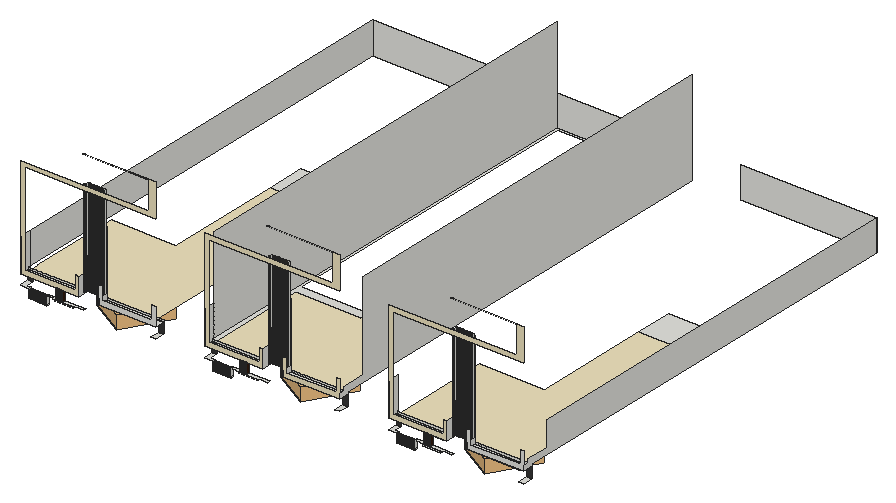
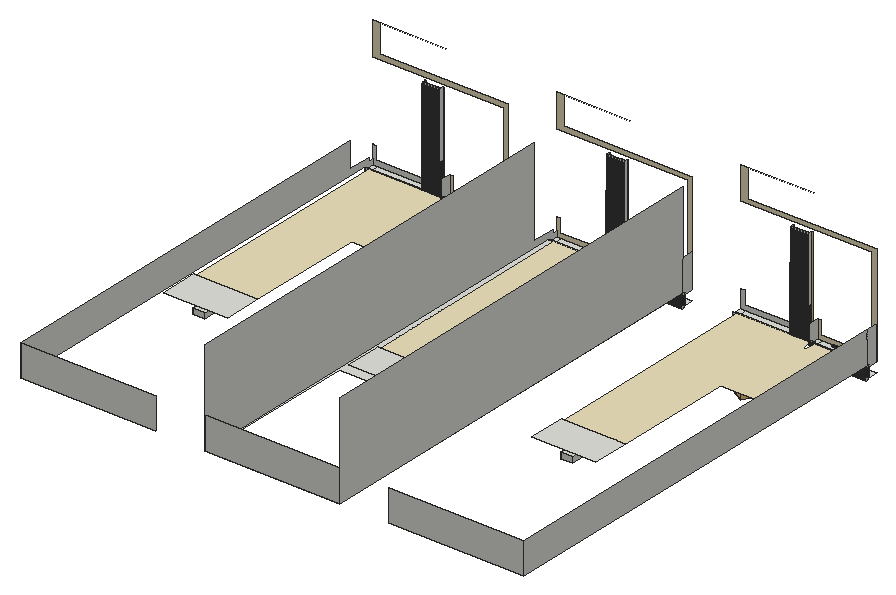
# SketchUp Ruby script. Lengths in inches.
U = 1.inch
M = Sketchup.active_model
def pt(a) = Geom::Point3d.new(a.map { |v| v * U })
def face(e, loops, mat)
  f = e.add_face(loops[0].map { |a| pt(a) })
  loops[1..].each { |l| e.add_face(l.map { |a| pt(a) }).erase! }
  f.material = f.back_material = mat if mat
  f
end
# faces: each face lists its corners as indices into pts; further lists are holes
def faces(e, pts, list, mat = nil) = list.each { |f| face(e, (f[0].is_a?(Array) ? f : [f]).map { |l| l.map { |i| pts[i] } }, mat) }
# xy, xz, yz: faces in a plane at the given z, y or x. An outline is a flat list of corners, or four numbers for a rectangle; further outlines are holes
def ring(l) = l.size == 4 ? [[l[0], l[1]], [l[2], l[1]], [l[2], l[3]], [l[0], l[3]]] : l.each_slice(2).to_a
def flat(e, list, mat, &to3) = list.each { |f| face(e, (f[0].is_a?(Array) ? f : [f]).map { |l| ring(l).map { |u, v| to3.(u, v) } }, mat) }
def xy(e, z, list, mat = nil) = flat(e, list, mat) { |x, y| [x, y, z] }
def xz(e, y, list, mat = nil) = flat(e, list, mat) { |x, z| [x, y, z] }
def yz(e, x, list, mat = nil) = flat(e, list, mat) { |y, z| [x, y, z] }
def lines(e, pts, list) = list.each { |a, b| e.add_line(pt(pts[a]), pt(pts[b])) }
# prism: a flat outline (further loops are holes) pulled along v
def prism(e, loops, v, mat = nil)
  f = face(e, loops, mat); d = Geom::Vector3d.new(v.map { |x| x * U })
  f.pushpull(f.normal.samedirection?(d) ? d.length : -d.length)
end
def box(e, o, s, mat = nil) = prism(e, [[o, [o[0] + s[0], o[1], o[2]], [o[0] + s[0], o[1] + s[1], o[2]], [o[0], o[1] + s[1], o[2]]]], [0, 0, s[2]], mat)
def at(x, y, z, deg = 0) = Geom::Transformation.translation(pt([x, y, z])) * Geom::Transformation.rotation(ORIGIN, Z_AXIS, deg.degrees)
def axes(o, x, y, z) = Geom::Transformation.new([*x, 0, *y, 0, *z, 0, *pt(o).to_a, 1])
def part(name) = M.definitions.add(name)
# library, detail: a bought-in or finely detailed component or shape, given as its bounding box
def library(name, o, s) = part(name).tap { |d| box(d.entities, o, s) }
def detail(e, o, s) = box(e.add_group.entities, o, s)
def put(e, d, t, mat = nil) = e.add_instance(d, t).tap { |i| i.material = mat if mat }
def group(e, t, mat = nil) = e.add_group.tap { |g| g.transformation = t; g.material = mat if mat }.entities
root = M.entities
M.materials.add("[Color D01]").color = [237, 225, 189]
M.materials.add("[Slate Light Tile]").color = [54, 54, 54]
M.materials.add("[Slate]").color = [102, 110, 108]
M.materials.add("[Wood Veneer 01]").color = [51, 28, 15]
c1 = library("002+Bmw+M4+++mat3.4+2017",[-252.8,19.48,9.01],[196.94,171.32,55.15])
c2 = library("Group\#1",[-0.5,-0.5,0],[4.42,1,384])
c3 = library("Group\#4",[-0.5,-0.5,0],[4.42,1,384])
xy(root,44.76,[[115.73,246.64,188.54,248.89],[849.29,246.64,922.1,248.89],[1582.85,246.64,1655.66,248.89],[115.73,248.89,188.54,254.15],[188.54,248.89,190.1,254.15],
  [849.29,248.89,922.1,254.15],[922.1,248.89,923.66,254.15],[1582.85,248.89,1655.66,254.15],[1655.66,248.89,1657.23,254.15],[115.73,254.15,188.54,255.71],
  [849.29,254.15,922.1,255.71],[1582.85,254.15,1655.66,255.71]])
xy(root,47.875,[[115.73,248.89,190.1,254.15],[849.29,248.89,923.66,254.15],[1582.85,248.89,1657.23,254.15]])
xy(root,50.625,[[115.73,248.89,188.54,254.15],[849.29,248.89,922.1,254.15],[1582.85,248.89,1655.66,254.15]])
xy(root,53.875,[[115.73,248.89,188.54,254.15],[849.29,248.89,922.1,254.15],[1582.85,248.89,1655.66,254.15]])
xy(root,56.625,[[115.73,248.89,188.54,254.15],[849.29,248.89,922.1,254.15],[1582.85,248.89,1655.66,254.15]])
xy(root,59.875,[[115.73,248.89,188.54,254.15],[849.29,248.89,922.1,254.15],[1582.85,248.89,1655.66,254.15]])
xy(root,62.625,[[115.73,248.89,188.54,254.15],[849.29,248.89,922.1,254.15],[1582.85,248.89,1655.66,254.15]])
xy(root,65.875,[[115.73,248.89,188.54,254.15],[849.29,248.89,922.1,254.15],[1582.85,248.89,1655.66,254.15]])
xy(root,68.625,[[115.73,248.89,188.54,254.15],[849.29,248.89,922.1,254.15],[1582.85,248.89,1655.66,254.15]])
xy(root,71.875,[[115.73,248.89,188.54,254.15],[849.29,248.89,922.1,254.15],[1582.85,248.89,1655.66,254.15]])
xy(root,74.24,[[224.55,243.46,295.95,246.64],[958.11,243.46,1029.51,246.64],[1691.68,243.46,1763.07,246.64]])
xy(root,74.625,[[115.73,248.89,188.54,254.15],[849.29,248.89,922.1,254.15],[1582.85,248.89,1655.66,254.15]])
xy(root,76.4375,[[603.24,246.64,622,286.21],[1336.8,246.64,1355.5625,286.21],[2070.36,246.64,2089.125,286.21]])
xy(root,77.875,[[115.73,248.89,188.54,254.15],[849.29,248.89,922.1,254.15],[1582.85,248.89,1655.66,254.15]])
xy(root,79.95,[[215.84,243.46,224.54,243.46,224.54,255.71,188.54,255.71,188.54,246.64,215.84,246.64],[224.54,243.46,230.14,246.64],[230.14,243.46,235.97,246.64],[235.97,243.46,241.57,246.64],[241.57,243.46,248.39,246.64],
  [248.39,243.46,253.99,246.64],[253.99,243.46,303.85,243.46,303.85,246.64,337.76,246.64,337.76,255.71,253.99,255.71],[949.4,243.46,958.1,243.46,958.1,255.71,922.1,255.71,922.1,246.64,949.4,246.64],[958.1,243.46,963.7,246.64],[963.7,243.46,969.54,246.64],
  [969.54,243.46,975.14,246.64],[975.14,243.46,981.95,246.64],[981.95,243.46,987.55,246.64],[987.55,243.46,1037.42,243.46,1037.42,246.64,1071.32,246.64,1071.32,255.71,987.55,255.71],[1682.97,243.46,1691.67,243.46,1691.67,255.71,1655.66,255.71,1655.66,246.64,1682.97,246.64],
  [1691.67,243.46,1697.27,246.64],[1697.27,243.46,1703.1,246.64],[1703.1,243.46,1708.7,246.64],[1708.7,243.46,1715.51,246.64],[1715.51,243.46,1721.11,246.64],
  [1721.11,243.46,1770.98,243.46,1770.98,246.64,1804.89,246.64,1804.89,255.71,1721.11,255.71],[83.125,246.64,115.73,246.64,115.73,255.71,101.95,255.71,101.95,286.21,83.125,286.21],[230.14,246.64,235.97,255.71],[241.57,246.64,248.39,255.71],[816.6875,246.64,849.29,246.64,849.29,255.71,835.51,255.71,835.51,286.21,816.6875,286.21],
  [963.7,246.64,969.54,255.71],[975.14,246.64,981.95,255.71],[1550.25,246.64,1582.85,246.64,1582.85,255.71,1569.07,255.71,1569.07,286.21,1550.25,286.21],[1697.27,246.64,1703.1,255.71],[1708.7,246.64,1715.51,255.71]])
xy(root,79.95,[[224.54,246.64,230.14,255.71],[235.97,246.64,241.57,255.71],[248.39,246.64,253.99,255.71],[958.1,246.64,963.7,255.71],[969.54,246.64,975.14,255.71],
  [981.95,246.64,987.55,255.71],[1691.67,246.64,1697.27,255.71],[1703.1,246.64,1708.7,255.71],[1715.51,246.64,1721.11,255.71]],"[Wood Veneer 01]")
xy(root,91.5625,[[452.08,1150.15,500.08,1298.96],[1185.65,1150.15,1233.65,1298.96],[1919.21,1150.15,1967.21,1298.96]])
xy(root,114.3125,[[452.08,1150.15,500.08,1298.96],[1185.65,1150.15,1233.65,1298.96],[1919.21,1150.15,1967.21,1298.96]])
xy(root,120.375,[[83.125,246.64,83.125,286.21,298.48,286.21,298.48,246.64,253.99,246.64,253.99,255.71,248.39,255.71,248.39,246.64,241.57,246.64,241.57,255.71,235.97,255.71,235.97,246.64,230.14,246.64,230.14,255.71,224.54,255.71,224.54,246.64],[298.48,246.64,315.43,286.21],[396.57,246.64,603.24,286.21],[603.24,246.64,622,286.21],[816.6875,246.64,816.6875,286.21,1032.04,286.21,1032.04,246.64,987.55,246.64,987.55,255.71,981.95,255.71,981.95,246.64,975.14,246.64,975.14,255.71,969.54,255.71,969.54,246.64,963.7,246.64,963.7,255.71,958.1,255.71,958.1,246.64],
  [1032.04,246.64,1049,286.21],[1130.14,246.64,1336.8,286.21],[1336.8,246.64,1355.5625,286.21],[1550.25,246.64,1550.25,286.21,1765.6,286.21,1765.6,246.64,1721.11,246.64,1721.11,255.71,1715.51,255.71,1715.51,246.64,1708.7,246.64,1708.7,255.71,1703.1,255.71,1703.1,246.64,1697.27,246.64,1697.27,255.71,1691.67,255.71,1691.67,246.64],[1765.6,246.64,1782.56,286.21],
  [1863.7,246.64,2070.36,286.21],[2070.36,246.64,2089.125,286.21],[83.125,286.21,298.48,293.46],[298.48,286.21,315.43,293.46],[816.6875,286.21,1032.04,293.46],
  [1032.04,286.21,1049,293.46],[1550.25,286.21,1765.6,293.46],[1765.6,286.21,1782.56,293.46]])
xy(root,128.6875,[[[816.6875,286.21,816.6875,2003.89,1355.5625,2003.89,1355.5625,286.21,1336.8,286.21,1336.8,1150.15,1346.93,1150.15,1346.93,1298.96,1092.25,1298.96,1092.25,679.27,833.39,679.27,833.39,310.87,835.51,310.87,835.51,286.21],[825.32,714.9,1077.64,714.9,1077.64,1340.4,1346.93,1340.4,1346.93,1995.26,825.32,1995.26]],[358.6875,1150.15,613.36,1298.96],[1092.25,1150.15,1346.93,1298.96],[1825.8125,1150.15,2080.49,1298.96]])
xy(root,128.6875,[[[318.81,271.96,318.81,286.21,101.95,286.21,101.95,310.87,99.82,310.87,99.82,679.27,358.6875,679.27,358.6875,1150.15,603.24,1150.15,603.24,286.21,393.55,286.21,393.55,272.89,390.12,272.89,390.12,286.21,388.23,286.21,388.23,283.46,384.81,283.46,384.81,286.21,382.23,286.21,382.23,283.46,378.81,283.46,378.81,286.21,376.23,286.21,376.23,283.46,372.81,283.46,372.81,286.21,370.23,286.21,370.23,283.46,366.81,283.46,366.81,286.21,364.23,286.21,364.23,283.46,360.81,283.46,360.81,286.21,358.23,286.21,358.23,283.46,354.81,283.46,354.81,286.21,352.23,286.21,352.23,283.46,348.81,283.46,348.81,286.21,346.23,286.21,346.23,282.52,342.81,282.52,342.81,286.21,340.23,286.21,340.23,282.52,336.81,282.52,336.81,286.21,334.23,286.21,334.23,282.52,330.81,282.52,330.81,286.21,328.23,286.21,328.23,282.52,324.81,282.52,324.81,286.21,322.23,286.21,322.23,271.96],[294.56,294.84,310.12,329.78]],[[1052.37,271.96,1052.37,286.21,835.51,286.21,835.51,310.87,833.39,310.87,833.39,679.27,1092.25,679.27,1092.25,1150.15,1336.8,1150.15,1336.8,286.21,1127.11,286.21,1127.11,272.89,1123.68,272.89,1123.68,286.21,1121.8,286.21,1121.8,283.46,1118.37,283.46,1118.37,286.21,1115.8,286.21,1115.8,283.46,1112.37,283.46,1112.37,286.21,1109.8,286.21,1109.8,283.46,1106.37,283.46,1106.37,286.21,1103.8,286.21,1103.8,283.46,1100.37,283.46,1100.37,286.21,1097.8,286.21,1097.8,283.46,1094.37,283.46,1094.37,286.21,1091.8,286.21,1091.8,283.46,1088.37,283.46,1088.37,286.21,1085.8,286.21,1085.8,283.46,1082.37,283.46,1082.37,286.21,1079.8,286.21,1079.8,282.52,1076.37,282.52,1076.37,286.21,1073.8,286.21,1073.8,282.52,1070.37,282.52,1070.37,286.21,1067.8,286.21,1067.8,282.52,1064.37,282.52,1064.37,286.21,1061.8,286.21,1061.8,282.52,1058.37,282.52,1058.37,286.21,1055.8,286.21,1055.8,271.96],[1028.12,294.84,1043.68,329.78]],[[1785.93,271.96,1785.93,286.21,1569.07,286.21,1569.07,310.87,1566.95,310.87,1566.95,679.27,1825.8125,679.27,1825.8125,1150.15,2070.36,1150.15,2070.36,286.21,1860.67,286.21,1860.67,272.89,1857.25,272.89,1857.25,286.21,1855.36,286.21,1855.36,283.46,1851.93,283.46,1851.93,286.21,1849.36,286.21,1849.36,283.46,1845.93,283.46,1845.93,286.21,1843.36,286.21,1843.36,283.46,1839.93,283.46,1839.93,286.21,1837.36,286.21,1837.36,283.46,1833.93,283.46,1833.93,286.21,1831.36,286.21,1831.36,283.46,1827.93,283.46,1827.93,286.21,1825.36,286.21,1825.36,283.46,1821.93,283.46,1821.93,286.21,1819.36,286.21,1819.36,283.46,1815.93,283.46,1815.93,286.21,1813.36,286.21,1813.36,282.52,1809.93,282.52,1809.93,286.21,1807.36,286.21,1807.36,282.52,1803.93,282.52,1803.93,286.21,1801.36,286.21,1801.36,282.52,1797.93,282.52,1797.93,286.21,1795.36,286.21,1795.36,282.52,1791.93,282.52,1791.93,286.21,1789.36,286.21,1789.36,271.96],[1761.68,294.84,1777.24,329.78]]],"[Color D01]")
xz(root,246.64,[[396.57,120.375,622,120.375,622,193,609.07,193,609.07,140.625,409.32,140.625,409.32,193,396.57,193],[1863.7,120.375,2089.125,120.375,2089.125,193,2076.2,193,2076.2,140.625,1876.45,140.625,1876.45,193,1863.7,193]])
xz(root,246.64,[[83.125,120.375,315.43,120.375,315.43,193,303.35,193,303.35,140.625,100.18,140.625,100.18,506.8125,622,506.8125,622,636.53,330.81,636.53,330.81,635.84,593.4375,635.84,593.4375,524.9375,83.125,524.9375],[816.6875,120.375,1049,120.375,1049,193,1036.91,193,1036.91,140.625,833.74,140.625,833.74,506.8125,1355.5625,506.8125,1355.5625,636.53,1064.37,636.53,1064.37,635.84,1327,635.84,1327,524.9375,816.6875,524.9375],[1130.14,120.375,1355.5625,120.375,1355.5625,193,1342.64,193,1342.64,140.625,1142.89,140.625,1142.89,193,1130.14,193],[1550.25,120.375,1782.56,120.375,1782.56,193,1770.48,193,1770.48,140.625,1567.3,140.625,1567.3,506.8125,2089.125,506.8125,2089.125,636.53,1797.93,636.53,1797.93,635.84,2060.5625,635.84,2060.5625,524.9375,1550.25,524.9375]],"[Color D01]")
xz(root,246.64,[[230.14,79.95,235.97,120.375],[241.57,79.95,248.39,120.375],[963.7,79.95,969.54,120.375],[975.14,79.95,981.95,120.375],[1697.27,79.95,1703.1,120.375],
  [1708.7,79.95,1715.51,120.375]],"[Slate]")
xz(root,246.64,[[224.54,79.95,230.14,120.375],[235.97,79.95,241.57,120.375],[248.39,79.95,253.99,120.375],[958.1,79.95,963.7,120.375],[969.54,79.95,975.14,120.375],
  [981.95,79.95,987.55,120.375],[1691.67,79.95,1697.27,120.375],[1703.1,79.95,1708.7,120.375],[1715.51,79.95,1721.11,120.375]],"[Wood Veneer 01]")
xz(root,248.89,[[115.73,44.76,190.1,47.875],[849.29,44.76,923.66,47.875],[1582.85,44.76,1657.23,47.875],[115.73,50.625,188.54,53.875],[849.29,50.625,922.1,53.875],
  [1582.85,50.625,1655.66,53.875],[115.73,56.625,188.54,59.875],[849.29,56.625,922.1,59.875],[1582.85,56.625,1655.66,59.875],[115.73,62.625,188.54,65.875],
  [849.29,62.625,922.1,65.875],[1582.85,62.625,1655.66,65.875],[115.73,68.625,188.54,71.875],[849.29,68.625,922.1,71.875],[1582.85,68.625,1655.66,71.875],
  [115.73,74.625,188.54,77.875],[849.29,74.625,922.1,77.875],[1582.85,74.625,1655.66,77.875]])
xz(root,254.15,[[115.73,44.76,190.1,47.875],[849.29,44.76,923.66,47.875],[1582.85,44.76,1657.23,47.875],[115.73,50.625,188.54,53.875],[849.29,50.625,922.1,53.875],
  [1582.85,50.625,1655.66,53.875],[115.73,56.625,188.54,59.875],[849.29,56.625,922.1,59.875],[1582.85,56.625,1655.66,59.875],[115.73,62.625,188.54,65.875],
  [849.29,62.625,922.1,65.875],[1582.85,62.625,1655.66,65.875],[115.73,68.625,188.54,71.875],[849.29,68.625,922.1,71.875],[1582.85,68.625,1655.66,71.875],
  [115.73,74.625,188.54,77.875],[849.29,74.625,922.1,77.875],[1582.85,74.625,1655.66,77.875]])
xz(root,255.71,[[224.54,79.95,230.14,120.375],[235.97,79.95,241.57,120.375],[248.39,79.95,253.99,120.375],[958.1,79.95,963.7,120.375],[969.54,79.95,975.14,120.375],
  [981.95,79.95,987.55,120.375],[1691.67,79.95,1697.27,120.375],[1703.1,79.95,1708.7,120.375],[1715.51,79.95,1721.11,120.375]],"[Wood Veneer 01]")
xz(root,282.52,[[324.81,128.6875,328.23,512.6875],[330.81,128.6875,334.23,512.6875],[336.81,128.6875,340.23,512.6875],[342.81,128.6875,346.23,512.6875],[1058.37,128.6875,1061.8,512.6875],
  [1064.37,128.6875,1067.8,512.6875],[1070.37,128.6875,1073.8,512.6875],[1076.37,128.6875,1079.8,512.6875],[1791.93,128.6875,1795.36,512.6875],[1797.93,128.6875,1801.36,512.6875],
  [1803.93,128.6875,1807.36,512.6875],[1809.93,128.6875,1813.36,512.6875]],"[Wood Veneer 01]")
xz(root,283.46,[[348.81,128.6875,352.23,512.6875],[354.81,128.6875,358.23,512.6875],[360.81,128.6875,364.23,512.6875],[366.81,128.6875,370.23,512.6875],[372.81,128.6875,376.23,512.6875],
  [378.81,128.6875,382.23,512.6875],[384.81,128.6875,388.23,512.6875],[1082.37,128.6875,1085.8,512.6875],[1088.37,128.6875,1091.8,512.6875],[1094.37,128.6875,1097.8,512.6875],
  [1100.37,128.6875,1103.8,512.6875],[1106.37,128.6875,1109.8,512.6875],[1112.37,128.6875,1115.8,512.6875],[1118.37,128.6875,1121.8,512.6875],[1815.93,128.6875,1819.36,512.6875],
  [1821.93,128.6875,1825.36,512.6875],[1827.93,128.6875,1831.36,512.6875],[1833.93,128.6875,1837.36,512.6875],[1839.93,128.6875,1843.36,512.6875],[1845.93,128.6875,1849.36,512.6875],
  [1851.93,128.6875,1855.36,512.6875]],"[Wood Veneer 01]")
xz(root,286.21,[[83.125,120.375,101.95,128.6875],[101.95,120.375,298.48,128.6875],[298.48,120.375,315.43,128.6875],[396.57,120.375,603.24,128.6875],[603.24,120.375,622,128.6875],
  [816.6875,120.375,835.51,128.6875],[835.51,120.375,1032.04,128.6875],[1032.04,120.375,1049,128.6875],[1130.14,120.375,1336.8,128.6875],[1336.8,120.375,1355.5625,128.6875],
  [1550.25,120.375,1569.07,128.6875],[1569.07,120.375,1765.6,128.6875],[1765.6,120.375,1782.56,128.6875],[1863.7,120.375,2070.36,128.6875],[2070.36,120.375,2089.125,128.6875],
  [298.48,128.6875,315.43,134.6875],[322.23,128.6875,324.81,505.3125],[328.23,128.6875,330.81,505.3125],[334.23,128.6875,336.81,505.3125],[340.23,128.6875,342.81,505.3125],
  [346.23,128.6875,348.81,505.3125],[352.23,128.6875,354.81,505.3125],[358.23,128.6875,360.81,505.3125],[364.23,128.6875,366.81,505.3125],[370.23,128.6875,372.81,505.3125],
  [376.23,128.6875,378.81,505.3125],[382.23,128.6875,384.81,505.3125],[388.23,128.6875,390.12,505.3125],[393.55,128.6875,393.95,505.3125],[1032.04,128.6875,1049,134.6875],
  [1055.8,128.6875,1058.37,505.3125],[1061.8,128.6875,1064.37,505.3125],[1067.8,128.6875,1070.37,505.3125],[1073.8,128.6875,1076.37,505.3125],[1079.8,128.6875,1082.37,505.3125],
  [1085.8,128.6875,1088.37,505.3125],[1091.8,128.6875,1094.37,505.3125],[1097.8,128.6875,1100.37,505.3125],[1103.8,128.6875,1106.37,505.3125],[1109.8,128.6875,1112.37,505.3125],
  [1115.8,128.6875,1118.37,505.3125],[1121.8,128.6875,1123.68,505.3125],[1127.11,128.6875,1127.51,505.3125],[1765.6,128.6875,1782.56,134.6875],[1789.36,128.6875,1791.93,505.3125],
  [1795.36,128.6875,1797.93,505.3125],[1801.36,128.6875,1803.93,505.3125],[1807.36,128.6875,1809.93,505.3125],[1813.36,128.6875,1815.93,505.3125],[1819.36,128.6875,1821.93,505.3125],
  [1825.36,128.6875,1827.93,505.3125],[1831.36,128.6875,1833.93,505.3125],[1837.36,128.6875,1839.93,505.3125],[1843.36,128.6875,1845.93,505.3125],[1849.36,128.6875,1851.93,505.3125],
  [1855.36,128.6875,1857.25,505.3125],[1860.67,128.6875,1861.07,505.3125]])
xz(root,286.21,[[603.24,76.4375,622,120.375],[1336.8,76.4375,1355.5625,120.375],[2070.36,76.4375,2089.125,120.375],[83.125,79.95,101.95,120.375],[816.6875,79.95,835.51,120.375],
  [1550.25,79.95,1569.07,120.375]],"[Slate Light Tile]")
xz(root,286.21,[[315.43,128.6875,318.81,254.6875],[393.95,128.6875,396.57,380.6875],[1049,128.6875,1052.37,254.6875],[1127.51,128.6875,1130.14,380.6875],[1782.56,128.6875,1785.93,254.6875],
  [1861.07,128.6875,1863.7,380.6875]],"[Wood Veneer 01]")
xz(root,1150.15,[[452.08,91.5625,500.08,114.3125],[1185.65,91.5625,1233.65,114.3125],[1919.21,91.5625,1967.21,114.3125]],"[Wood Veneer 01]")
xz(root,1298.96,[[452.08,91.5625,500.08,114.3125],[1185.65,91.5625,1233.65,114.3125],[1919.21,91.5625,1967.21,114.3125]])
xz(root,2003.89,[[83.125,128.6875,622,254.6875],[816.6875,128.6875,1355.5625,254.6875],[1550.25,128.6875,2089.125,254.6875]])
yz(root,83.125,[[246.64,120.375,246.64,254.6875,293.46,254.6875,293.46,128.6875,286.21,128.6875,286.21,120.375],[286.21,120.375,293.46,128.6875],[293.46,128.6875,2003.89,254.6875]])
yz(root,115.73,[[248.89,44.625,254.15,44.76],[[246.64,44.76,248.89,44.76,248.89,47.875,254.15,47.875,254.15,44.76,255.71,44.76,255.71,79.95,246.64,79.95],[248.89,62.625,254.15,65.875],[248.89,74.625,254.15,77.875],[248.89,68.625,254.15,71.875],[248.89,56.625,254.15,59.875],[248.89,50.625,254.15,53.875]]])
yz(root,188.54,[[[246.64,44.76,255.71,79.95],[248.89,62.625,254.15,65.875],[248.89,74.625,254.15,77.875],[248.89,68.625,254.15,71.875],[248.89,56.625,254.15,59.875],[248.89,50.625,254.15,53.875]]])
yz(root,190.1,[[248.89,44.76,254.15,47.875]])
yz(root,224.54,[[246.64,79.95,255.71,120.375]],"[Wood Veneer 01]")
yz(root,230.14,[[246.64,79.95,255.71,120.375]],"[Wood Veneer 01]")
yz(root,235.97,[[246.64,79.95,255.71,120.375]],"[Wood Veneer 01]")
yz(root,241.57,[[246.64,79.95,255.71,120.375]],"[Wood Veneer 01]")
yz(root,248.39,[[246.64,79.95,255.71,120.375]],"[Wood Veneer 01]")
yz(root,253.99,[[246.64,79.95,255.71,120.375]],"[Wood Veneer 01]")
yz(root,315.43,[[246.64,120.375,286.21,193],[286.21,120.375,293.46,134.6875]])
yz(root,318.81,[[271.96,128.6875,286.21,254.6875]])
yz(root,322.23,[[271.96,128.6875,286.21,512.6875]])
yz(root,324.81,[[282.52,128.6875,286.21,254.6875]])
yz(root,328.23,[[282.52,128.6875,286.21,512.6875]])
yz(root,330.81,[[282.52,128.6875,286.21,254.6875]])
yz(root,334.23,[[282.52,128.6875,286.21,512.6875]])
yz(root,336.81,[[282.52,128.6875,286.21,254.6875]])
yz(root,340.23,[[282.52,128.6875,286.21,512.6875]])
yz(root,342.81,[[282.52,128.6875,286.21,254.6875]])
yz(root,346.23,[[282.52,128.6875,286.21,512.6875]])
yz(root,348.81,[[283.46,128.6875,286.21,254.6875]])
yz(root,352.23,[[283.46,128.6875,286.21,512.6875]])
yz(root,354.81,[[283.46,128.6875,286.21,254.6875]])
yz(root,358.23,[[283.46,128.6875,286.21,512.6875]])
yz(root,360.81,[[283.46,128.6875,286.21,254.6875]])
yz(root,364.23,[[283.46,128.6875,286.21,512.6875]])
yz(root,366.81,[[283.46,128.6875,286.21,254.6875]])
yz(root,370.23,[[283.46,128.6875,286.21,512.6875]])
yz(root,372.81,[[283.46,128.6875,286.21,254.6875]])
yz(root,376.23,[[283.46,128.6875,286.21,512.6875]])
yz(root,378.81,[[283.46,128.6875,286.21,254.6875]])
yz(root,382.23,[[283.46,128.6875,286.21,512.6875]])
yz(root,384.81,[[283.46,128.6875,286.21,254.6875]])
yz(root,388.23,[[283.46,128.6875,286.21,512.6875]])
yz(root,390.12,[[272.89,128.6875,286.21,254.6875]])
yz(root,393.55,[[272.89,128.6875,286.21,512.6875]])
yz(root,396.57,[[246.64,120.375,286.21,141.6875]])
yz(root,452.08,[[1150.15,91.5625,1298.96,114.3125]])
yz(root,500.08,[[1150.15,91.5625,1298.96,114.3125]])
yz(root,816.6875,[[246.64,120.375,246.64,254.6875,293.46,254.6875,293.46,128.6875,286.21,128.6875,286.21,120.375],[286.21,120.375,293.46,128.6875],[293.46,128.6875,2003.89,506.6875]])
yz(root,849.29,[[248.89,44.625,254.15,44.76],[[246.64,44.76,248.89,44.76,248.89,47.875,254.15,47.875,254.15,44.76,255.71,44.76,255.71,79.95,246.64,79.95],[248.89,74.625,254.15,77.875],[248.89,68.625,254.15,71.875],[248.89,62.625,254.15,65.875],[248.89,56.625,254.15,59.875],[248.89,50.625,254.15,53.875]]])
yz(root,922.1,[[[246.64,44.76,255.71,79.95],[248.89,74.625,254.15,77.875],[248.89,68.625,254.15,71.875],[248.89,62.625,254.15,65.875],[248.89,56.625,254.15,59.875],[248.89,50.625,254.15,53.875]]])
yz(root,923.66,[[248.89,44.76,254.15,47.875]])
yz(root,958.1,[[246.64,79.95,255.71,120.375]],"[Wood Veneer 01]")
yz(root,963.7,[[246.64,79.95,255.71,120.375]],"[Wood Veneer 01]")
yz(root,969.54,[[246.64,79.95,255.71,120.375]],"[Wood Veneer 01]")
yz(root,975.14,[[246.64,79.95,255.71,120.375]],"[Wood Veneer 01]")
yz(root,981.95,[[246.64,79.95,255.71,120.375]],"[Wood Veneer 01]")
yz(root,987.55,[[246.64,79.95,255.71,120.375]],"[Wood Veneer 01]")
yz(root,1049,[[246.64,120.375,286.21,193],[286.21,120.375,293.46,134.6875]])
yz(root,1052.37,[[271.96,128.6875,286.21,254.6875]])
yz(root,1055.8,[[271.96,128.6875,286.21,512.6875]])
yz(root,1058.37,[[282.52,128.6875,286.21,254.6875]])
yz(root,1061.8,[[282.52,128.6875,286.21,512.6875]])
yz(root,1064.37,[[282.52,128.6875,286.21,254.6875]])
yz(root,1067.8,[[282.52,128.6875,286.21,512.6875]])
yz(root,1070.37,[[282.52,128.6875,286.21,254.6875]])
yz(root,1073.8,[[282.52,128.6875,286.21,512.6875]])
yz(root,1076.37,[[282.52,128.6875,286.21,254.6875]])
yz(root,1079.8,[[282.52,128.6875,286.21,512.6875]])
yz(root,1082.37,[[283.46,128.6875,286.21,254.6875]])
yz(root,1085.8,[[283.46,128.6875,286.21,512.6875]])
yz(root,1088.37,[[283.46,128.6875,286.21,254.6875]])
yz(root,1091.8,[[283.46,128.6875,286.21,512.6875]])
yz(root,1094.37,[[283.46,128.6875,286.21,254.6875]])
yz(root,1097.8,[[283.46,128.6875,286.21,512.6875]])
yz(root,1100.37,[[283.46,128.6875,286.21,254.6875]])
yz(root,1103.8,[[283.46,128.6875,286.21,512.6875]])
yz(root,1106.37,[[283.46,128.6875,286.21,254.6875]])
yz(root,1109.8,[[283.46,128.6875,286.21,512.6875]])
yz(root,1112.37,[[283.46,128.6875,286.21,254.6875]])
yz(root,1115.8,[[283.46,128.6875,286.21,512.6875]])
yz(root,1118.37,[[283.46,128.6875,286.21,254.6875]])
yz(root,1121.8,[[283.46,128.6875,286.21,512.6875]])
yz(root,1123.68,[[272.89,128.6875,286.21,254.6875]])
yz(root,1127.11,[[272.89,128.6875,286.21,512.6875]])
yz(root,1130.14,[[246.64,120.375,286.21,141.6875]])
yz(root,1185.65,[[1150.15,91.5625,1298.96,114.3125]])
yz(root,1233.65,[[1150.15,91.5625,1298.96,114.3125]])
yz(root,1355.5625,[[246.64,120.375,286.21,120.375,286.21,128.6875,2003.89,128.6875,2003.89,506.6875,361.27,506.6875,361.27,154.75,266.43,154.75,266.43,140.625,246.64,140.625]])
yz(root,1550.25,[[246.64,120.375,246.64,254.6875,293.46,254.6875,293.46,128.6875,286.21,128.6875,286.21,120.375],[286.21,120.375,293.46,128.6875]])
yz(root,1582.85,[[248.89,44.625,254.15,44.76],[[246.64,44.76,248.89,44.76,248.89,47.875,254.15,47.875,254.15,44.76,255.71,44.76,255.71,79.95,246.64,79.95],[248.89,74.625,254.15,77.875],[248.89,68.625,254.15,71.875],[248.89,62.625,254.15,65.875],[248.89,56.625,254.15,59.875],[248.89,50.625,254.15,53.875]]])
yz(root,1655.66,[[[246.64,44.76,255.71,79.95],[248.89,74.625,254.15,77.875],[248.89,68.625,254.15,71.875],[248.89,62.625,254.15,65.875],[248.89,56.625,254.15,59.875],[248.89,50.625,254.15,53.875]]])
yz(root,1657.23,[[248.89,44.76,254.15,47.875]])
yz(root,1691.67,[[246.64,79.95,255.71,120.375]],"[Wood Veneer 01]")
yz(root,1697.27,[[246.64,79.95,255.71,120.375]],"[Wood Veneer 01]")
yz(root,1703.1,[[246.64,79.95,255.71,120.375]],"[Wood Veneer 01]")
yz(root,1708.7,[[246.64,79.95,255.71,120.375]],"[Wood Veneer 01]")
yz(root,1715.51,[[246.64,79.95,255.71,120.375]],"[Wood Veneer 01]")
yz(root,1721.11,[[246.64,79.95,255.71,120.375]],"[Wood Veneer 01]")
yz(root,1782.56,[[246.64,120.375,286.21,193],[286.21,120.375,293.46,134.6875]])
yz(root,1785.93,[[271.96,128.6875,286.21,254.6875]])
yz(root,1789.36,[[271.96,128.6875,286.21,512.6875]])
yz(root,1791.93,[[282.52,128.6875,286.21,254.6875]])
yz(root,1795.36,[[282.52,128.6875,286.21,512.6875]])
yz(root,1797.93,[[282.52,128.6875,286.21,254.6875]])
yz(root,1801.36,[[282.52,128.6875,286.21,512.6875]])
yz(root,1803.93,[[282.52,128.6875,286.21,254.6875]])
yz(root,1807.36,[[282.52,128.6875,286.21,512.6875]])
yz(root,1809.93,[[282.52,128.6875,286.21,254.6875]])
yz(root,1813.36,[[282.52,128.6875,286.21,512.6875]])
yz(root,1815.93,[[283.46,128.6875,286.21,254.6875]])
yz(root,1819.36,[[283.46,128.6875,286.21,512.6875]])
yz(root,1821.93,[[283.46,128.6875,286.21,254.6875]])
yz(root,1825.36,[[283.46,128.6875,286.21,512.6875]])
yz(root,1827.93,[[283.46,128.6875,286.21,254.6875]])
yz(root,1831.36,[[283.46,128.6875,286.21,512.6875]])
yz(root,1833.93,[[283.46,128.6875,286.21,254.6875]])
yz(root,1837.36,[[283.46,128.6875,286.21,512.6875]])
yz(root,1839.93,[[283.46,128.6875,286.21,254.6875]])
yz(root,1843.36,[[283.46,128.6875,286.21,512.6875]])
yz(root,1845.93,[[283.46,128.6875,286.21,254.6875]])
yz(root,1849.36,[[283.46,128.6875,286.21,512.6875]])
yz(root,1851.93,[[283.46,128.6875,286.21,254.6875]])
yz(root,1855.36,[[283.46,128.6875,286.21,512.6875]])
yz(root,1857.25,[[272.89,128.6875,286.21,254.6875]])
yz(root,1860.67,[[272.89,128.6875,286.21,512.6875]])
yz(root,1863.7,[[246.64,120.375,286.21,141.6875]])
yz(root,1919.21,[[1150.15,91.5625,1298.96,114.3125]])
yz(root,1967.21,[[1150.15,91.5625,1298.96,114.3125]])
yz(root,2089.125,[[246.64,120.375,286.21,120.375,286.21,128.6875,2003.89,128.6875,2003.89,254.6875,361.27,254.6875,361.27,154.75,266.43,154.75,266.43,140.625,246.64,140.625]])
put(root,c1,at(1304.09,508.33,8.6875,60))
put(root,c1,at(2037.66,508.33,8.6875,60))
put(root,c1,at(570.53,508.33,8.6875,60))
put(root,c2,at(1052.37,271.96,128.6875))
put(root,c3,at(1123.68,272.89,128.6875))
put(root,c2,at(1785.93,271.96,128.6875))
put(root,c3,at(1857.25,272.89,128.6875))
put(root,c3,at(390.12,272.89,128.6875))
put(root,c2,at(318.81,271.96,128.6875))
